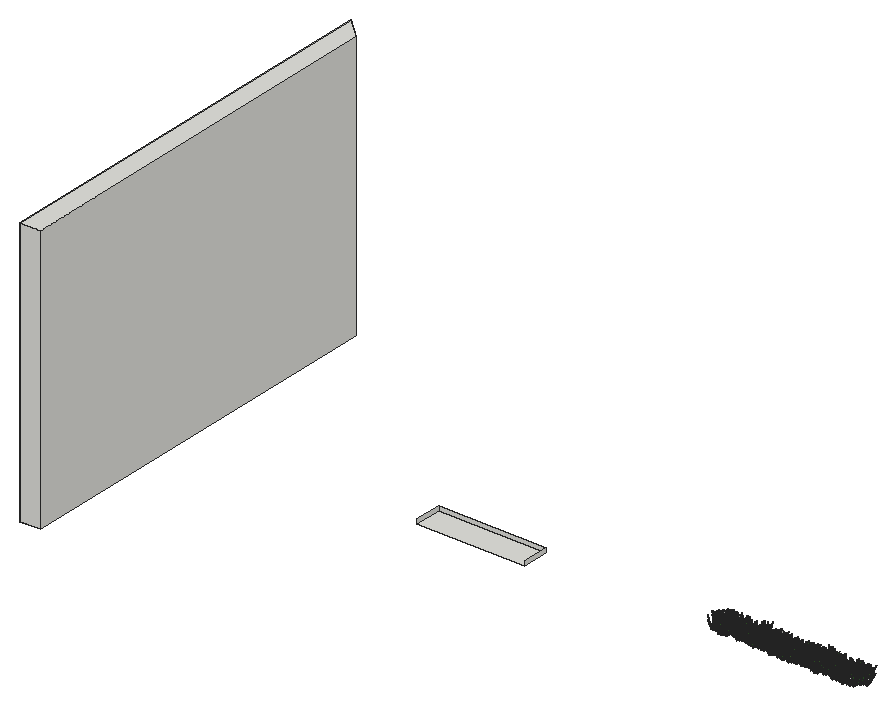
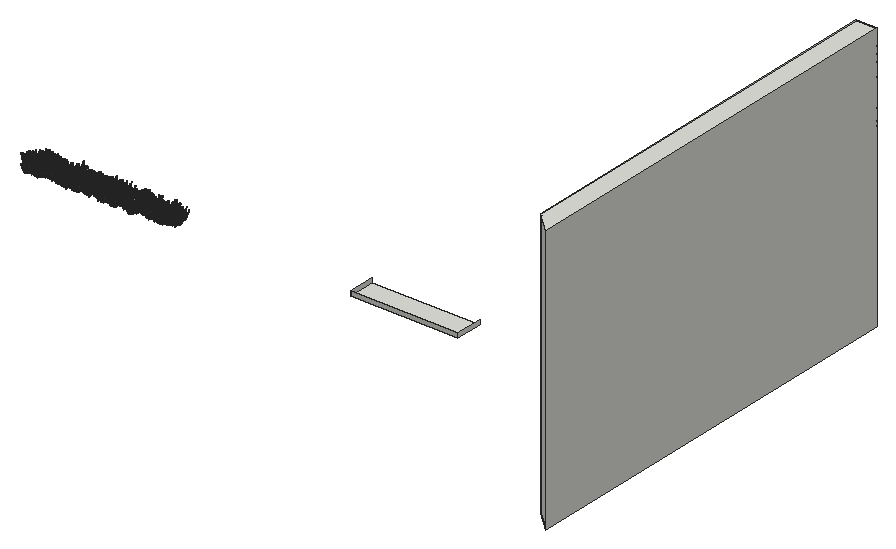
# SketchUp Ruby script. Lengths in inches.
U = 1.inch
M = Sketchup.active_model
def pt(a) = Geom::Point3d.new(a.map { |v| v * U })
def face(e, loops, mat)
  f = e.add_face(loops[0].map { |a| pt(a) })
  loops[1..].each { |l| e.add_face(l.map { |a| pt(a) }).erase! }
  f.material = f.back_material = mat if mat
  f
end
# faces: each face lists its corners as indices into pts; further lists are holes
def faces(e, pts, list, mat = nil) = list.each { |f| face(e, (f[0].is_a?(Array) ? f : [f]).map { |l| l.map { |i| pts[i] } }, mat) }
# xy, xz, yz: faces in a plane at the given z, y or x. An outline is a flat list of corners, or four numbers for a rectangle; further outlines are holes
def ring(l) = l.size == 4 ? [[l[0], l[1]], [l[2], l[1]], [l[2], l[3]], [l[0], l[3]]] : l.each_slice(2).to_a
def flat(e, list, mat, &to3) = list.each { |f| face(e, (f[0].is_a?(Array) ? f : [f]).map { |l| ring(l).map { |u, v| to3.(u, v) } }, mat) }
def xy(e, z, list, mat = nil) = flat(e, list, mat) { |x, y| [x, y, z] }
def xz(e, y, list, mat = nil) = flat(e, list, mat) { |x, z| [x, y, z] }
def yz(e, x, list, mat = nil) = flat(e, list, mat) { |y, z| [x, y, z] }
def lines(e, pts, list) = list.each { |a, b| e.add_line(pt(pts[a]), pt(pts[b])) }
# prism: a flat outline (further loops are holes) pulled along v
def prism(e, loops, v, mat = nil)
  f = face(e, loops, mat); d = Geom::Vector3d.new(v.map { |x| x * U })
  f.pushpull(f.normal.samedirection?(d) ? d.length : -d.length)
end
def box(e, o, s, mat = nil) = prism(e, [[o, [o[0] + s[0], o[1], o[2]], [o[0] + s[0], o[1] + s[1], o[2]], [o[0], o[1] + s[1], o[2]]]], [0, 0, s[2]], mat)
def at(x, y, z, deg = 0) = Geom::Transformation.translation(pt([x, y, z])) * Geom::Transformation.rotation(ORIGIN, Z_AXIS, deg.degrees)
def axes(o, x, y, z) = Geom::Transformation.new([*x, 0, *y, 0, *z, 0, *pt(o).to_a, 1])
def part(name) = M.definitions.add(name)
# library, detail: a bought-in or finely detailed component or shape, given as its bounding box
def library(name, o, s) = part(name).tap { |d| box(d.entities, o, s) }
def detail(e, o, s) = box(e.add_group.entities, o, s)
def put(e, d, t, mat = nil) = e.add_instance(d, t).tap { |i| i.material = mat if mat }
def group(e, t, mat = nil) = e.add_group.tap { |g| g.transformation = t; g.material = mat if mat }.entities
root = M.entities
M.materials.add("Material1").color = [58, 110, 58]
M.materials.add("Material10").color = [48, 100, 38]
M.materials.add("Material3").color = [68, 110, 58]
M.materials.add("Material4").color = [48, 90, 38]
M.materials.add("Material5").color = [68, 110, 48]
M.materials.add("Material6").color = [48, 90, 48]
M.materials.add("Material8").color = [58, 90, 38]
M.materials.add("Material9").color = [68, 100, 58]
c1 = part("grass00")
p = [[-0.6875,0.15,0],[-0.56,0.08,5.52],[-0.04,0.03,2.76],[0.48,-0.02,0],[0.35,-0.02,5.52],[-0.1,-0.14,5.52],
  [-0.12,0.65,8.37],[-0.42,0.65,8.37]]
faces(c1.entities,p,[[0,1,2,3],[3,2,4],[1,5,2],[5,4,2],[1,6,5],[4,5,6],[7,6,1]])
c2 = part("Group16\#1")
put(c2.entities,c1,axes([1.44,-0.61,-0.01],[0.05352,0.12609,0],[-0.10704,0.04543,0.07239],[0.06664,-0.02828,0.11628]),"Material6")
put(c2.entities,c1,axes([0.76,-0.15,-0.01],[0.04676,0.24062,0],[-0.23162,0.04501,0.06642],[0.0652,-0.01267,0.23595]),"Material3")
put(c2.entities,c1,axes([0.79,0.01,-0.01],[-0.00606,0.34651,0],[-0.34381,-0.00602,0.0432],[0.04319,0.00076,0.34386]))
put(c2.entities,c1,axes([1,0.23,-0.01],[-0.07192,0.31144,0],[-0.28722,-0.06632,0.1236],[0.12043,0.02781,0.29478]),"Material5")
put(c2.entities,c1,axes([1.66,0.77,-0.01],[-0.13828,0.29651,0],[-0.21551,-0.1005,0.22471],[0.20365,0.09498,0.23779]),"Material10")
put(c2.entities,c1,axes([0.6875,0.52,-0.01],[-0.18126,0.24051,0],[-0.22746,-0.17142,0.09788],[0.07817,0.05891,0.28481]),"Material5")
put(c2.entities,c1,axes([0.68,0.78,-0.01],[-0.215,0.18688,0],[-0.12385,-0.14248,0.21334],[0.13995,0.16101,0.18878]),"Material3")
put(c2.entities,c1,axes([0.56,1,-0.01],[-0.13756,0.07624,0],[-0.06159,-0.11112,0.0927],[0.04494,0.08108,0.12705]),"Material5")
put(c2.entities,c1,axes([0.2,0.64,-0.01],[-0.23729,0.07254,0],[-0.05711,-0.18681,0.153],[0.04473,0.14632,0.19535]),"Material10")
put(c2.entities,c1,axes([0.0625,0.72,-0.01],[-0.28874,0.02525,0],[-0.02179,-0.24916,0.14647],[0.01276,0.14591,0.25012]),"Material3")
put(c2.entities,c1,axes([-0.08,0.62,-0.01],[-0.34089,-0.04187,0],[0.03255,-0.26504,0.216],[-0.02633,0.21439,0.26703]),"Material10")
put(c2.entities,c1,axes([-0.34,0.98,-0.01],[-0.14314,-0.0493,0],[0.04397,-0.12769,0.06843],[-0.02228,0.0647,0.13505]),"Material10")
put(c2.entities,c1,axes([-0.87,1.45,-0.01],[-0.23488,-0.14114,0],[0.13761,-0.22901,0.06087],[-0.03135,0.05217,0.26717]))
put(c2.entities,c1,axes([-0.72,0.77,-0.01],[-0.14208,-0.13251,0],[0.07209,-0.0773,0.16301],[-0.11118,0.11922,0.1057]),"Material10")
put(c2.entities,c1,axes([-0.62,0.43,-0.01],[-0.14845,-0.21203,0],[0.18654,-0.13061,0.12304],[-0.10079,0.07057,0.22772]),"Material3")
put(c2.entities,c1,axes([-0.68,0.29,-0.01],[-0.13639,-0.32136,0],[0.31723,-0.13464,0.05579],[-0.05136,0.0218,0.34462]),"Material4")
put(c2.entities,c1,axes([-0.64,0.125,-0.01],[-0.0458,-0.23569,0],[0.22124,-0.043,0.08276],[-0.08124,0.01579,0.22538]),"Material1")
put(c2.entities,c1,axes([-1.6,-0.03,-0.01],[0.00576,-0.32897,0],[0.27526,0.00482,0.18018],[-0.18015,-0.00315,0.2753]),"Material5")
put(c2.entities,c1,axes([-1.36,-0.31,-0.01],[0.05718,-0.24765,0],[0.18172,0.04196,0.17267],[-0.16825,-0.03885,0.1865]),"Material10")
put(c2.entities,c1,axes([-1.54,-0.72,-0.01],[0.06537,-0.14017,0],[0.13555,0.06321,0.03939],[-0.0357,-0.01665,0.14956]))
put(c2.entities,c1,axes([-1.19,-0.9,-0.01],[0.09597,-0.12735,0],[0.11214,0.08451,0.07557],[-0.06035,-0.04548,0.14042]),"Material9")
put(c2.entities,c1,axes([-0.47,-0.54,-0.01],[0.11588,-0.10072,0],[0.0618,0.0711,0.12124],[-0.07953,-0.0915,0.0942]))
put(c2.entities,c1,axes([-0.47,-0.84,-0.01],[0.11927,-0.0661,0],[0.06603,0.11913,0.00646],[-0.00313,-0.00565,0.13621]),"Material5")
put(c2.entities,c1,axes([-0.38,-1.24,-0.01],[0.28037,-0.08571,0],[0.0618,0.20215,0.20315],[-0.05939,-0.19428,0.21139]),"Material9")
put(c2.entities,c1,axes([-0.06,-0.66,-0.01],[0.22719,-0.01987,0],[0.01247,0.14255,0.17758],[-0.01547,-0.17691,0.1431]),"Material8")
put(c2.entities,c1,axes([0.11,-0.89,-0.01],[0.14882,0.01828,0],[-0.01058,0.08611,0.12229],[0.01491,-0.12138,0.08676]),"Material6")
put(c2.entities,c1,axes([0.25,-0.72,-0.01],[0.20481,0.07053,0],[-0.06206,0.18022,0.10291],[0.03351,-0.0973,0.1906]),"Material6")
put(c2.entities,c1,axes([0.85,-1.42,-0.01],[0.16481,0.09904,0],[-0.09472,0.15762,0.05616],[0.02893,-0.04814,0.18389]),"Material5")
put(c2.entities,c1,axes([1.01,-1.09,-0.01],[0.21858,0.20385,0],[-0.17495,0.1876,0.15339],[0.10462,-0.11218,0.25652]),"Material10")
put(c2.entities,c1,axes([1.01,-0.71,-0.01],[0.08733,0.12473,0],[-0.06445,0.04512,0.13037],[0.1068,-0.07477,0.07867]),"Material6")
c3 = part("Group15\#1")
put(c3.entities,c2,at(0,0,0))
c4 = part("3darcstudiotree_grass00\#1")
put(c4.entities,c3,at(0,0,0))
xy(root,0,[[138.47,142.5,186.47,154.5]])
xz(root,154.5,[[138.47,0,186.47,2]])
yz(root,138.47,[[142.5,0,154.5,2]])
yz(root,186.47,[[142.5,0,154.5,2]])
put(root,c4,axes([328.01,147.54,0.25],[-0.99812,-0.23597,0],[0.29966,-0.87317,-0.03955],[0.01934,-0.05634,1.95202]))
put(root,c4,axes([303.16,147.6,0.25],[-0.99427,-0.5448,0],[0.56102,-0.70534,-0.0411],[0.03193,-0.04014,1.43569]))
put(root,c4,axes([325.42,147.52,0.25],[-1.23292,0.07319,0],[-0.09013,-1.04602,-0.06114],[-0.006,-0.06962,1.73764]))
put(root,c4,axes([329.43,147.77,0.25],[1.07781,0.18938,0],[-0.2093,0.82062,-0.03259],[-0.01079,0.04231,1.61556]))
put(root,c4,axes([293.99,147.58,0.25],[0.51316,0.9034,0],[-0.96575,0.37791,-0.03917],[-0.05959,0.02332,1.79585]))
put(root,c4,axes([321.9,147.76,0.25],[-0.54141,-0.69646,0],[0.787,-0.42147,-0.04434],[0.0525,-0.02812,1.31982]))
put(root,c4,axes([313.53,147.49,0.25],[-0.21956,0.99901,0],[-1.27509,-0.19305,-0.02378],[-0.03535,-0.00535,1.95907]))
put(root,c4,axes([298.41,147.61,0.25],[-0.29595,0.95829,0],[-1.17706,-0.25043,-0.05431],[-0.07294,-0.01552,1.6847]))
put(root,c4,axes([270.6875,147.76,0.25],[-0.64666,0.77516,0],[-0.79891,-0.45913,-0.03104],[-0.04689,-0.02695,1.78553]))
put(root,c4,axes([313.62,148.16,0.25],[1.22362,0.01748,0],[-0.01942,0.93658,-0.04862],[-0.00103,0.04974,1.39123]))
put(root,c4,axes([285.41,148.17,0.25],[-0.14791,-0.94502,0],[0.91047,-0.09817,-0.04034],[0.06426,-0.00693,1.47504]))
put(root,c4,axes([278.49,148.28,0.25],[-0.53102,-0.66775,0],[0.76975,-0.4217,-0.03406],[0.05336,-0.02923,1.73123]))
put(root,c4,axes([289.31,148.46,0.25],[0.95354,-0.47305,0],[0.61642,0.85599,-0.05659],[0.03982,0.0553,1.64805]))
put(root,c4,axes([317.27,148.26,0.25],[0.69662,0.57833,0],[-0.72973,0.60553,-0.04694],[-0.05459,0.0453,1.69685]))
put(root,c4,axes([283.84,148.47,0.25],[-0.01645,-0.79546,0],[1.12073,-0.01596,-0.0405],[0.06828,-0.00097,1.89003]))
put(root,c4,axes([307.7,148.16,0.25],[-0.67385,0.62223,0],[-0.80238,-0.59862,-0.05045],[-0.05166,-0.03854,1.48531]))
put(root,c4,axes([296.36,148.12,0.25],[-1.1835,0.3706,0],[-0.45111,-0.99242,-0.03096],[-0.01538,-0.03383,1.79846]))
put(root,c4,axes([283.37,148.31,0.25],[-0.12789,0.83027,0],[-1.23138,-0.13067,-0.0277],[-0.0416,-0.00441,1.87956]))
put(root,c4,axes([295.22,148.47,0.25],[0.68284,0.56041,0],[-0.63274,0.53112,-0.02576],[-0.03793,0.03184,1.88472]))
put(root,c4,axes([310.07,148.73,0.25],[0.39676,-0.79081,0],[0.95001,0.32835,-0.04485],[0.06401,0.02212,1.59096]))
put(root,c4,axes([322.74,148.87,0.25],[0.81664,-0.78547,0],[0.80725,0.57818,-0.04774],[0.06475,0.04638,1.91023]))
put(root,c4,axes([298.375,148.73,0.25],[0.72037,0.53225,0],[-0.78121,0.72839,-0.03405],[-0.03196,0.0298,1.65877]))
put(root,c4,axes([267.24,148.87,0.25],[1.1348,0.18325,0],[-0.22931,0.97826,-0.03864],[-0.01139,0.04857,1.85268]))
put(root,c4,axes([323.75,148.72,0.25],[0.82375,0.73045,0],[-0.83513,0.6488,-0.05678],[-0.04846,0.03764,1.337]))
put(root,c4,axes([287.74,148.83,0.25],[-0.54485,-0.78399,0],[0.98958,-0.47378,-0.05686],[0.05654,-0.02707,1.31145]))
put(root,c4,axes([327.1,148.96,0.25],[0.55568,-0.81643,0],[0.99319,0.46568,-0.05349],[0.08034,0.03767,1.96798]))
put(root,c4,axes([272.17,148.61,0.25],[-0.33702,0.82532,0],[-1.09541,-0.30816,-0.05878],[-0.06687,-0.01881,1.38915]))
put(root,c4,axes([312.09,149,0.25],[0.98512,-0.69325,0],[0.69961,0.68488,-0.04452],[0.05205,0.05095,1.95574]))
put(root,c4,axes([308.19,148.69,0.25],[0.10661,0.83198,0],[-1.11243,0.0982,-0.05804],[-0.07208,0.00636,1.39706]))
put(root,c4,axes([304.56,148.93,0.25],[-0.23365,-0.75886,0],[0.96416,-0.20451,-0.03508],[0.06527,-0.01385,1.91126]))
put(root,c4,axes([328.56,148.91,0.25],[-0.34662,-0.71179,0],[1.07984,-0.36226,-0.05241],[0.06977,-0.02341,1.67241]))
put(root,c4,axes([291.52,148.86,0.25],[-0.96963,-0.34021,0],[0.44355,-0.87089,-0.0473],[0.02319,-0.04554,1.43445]))
put(root,c4,axes([299.84,148.98,0.25],[0.68299,0.59104,0],[-0.74364,0.59199,-0.02632],[-0.036,0.02866,1.95302]))
put(root,c4,axes([325.33,148.93,0.25],[-0.68826,0.85119,0],[-0.91752,-0.51109,-0.03945],[-0.04757,-0.0265,1.6047]))
g1 = group(root,at(28.97,57,0))
prism(g1,[[[0,184.95,0],[9,176.76,0],[9,0,0],[0,0,0]]],[0,0,120])
put(root,c4,axes([294.65,149.54,0.25],[-0.53689,-0.61201,0],[0.94056,-0.56841,-0.06067],[0.0763,-0.04611,1.80988]))
put(root,c4,axes([309.77,149.41,0.25],[-1.07879,-0.10115,0],[0.14303,-1.0509,-0.03054],[0.00494,-0.03632,1.83699]))
put(root,c4,axes([299.68,149.43,0.25],[-1.04284,0.49546,0],[-0.47914,-0.69475,-0.03218],[-0.02748,-0.03984,1.65786]))
put(root,c4,axes([330.25,149.6,0.25],[1.09397,0.55734,0],[-0.51476,0.69606,-0.0354],[-0.03655,0.04943,1.94218]))
put(root,c4,axes([307.6,149.45,0.25],[-0.41932,0.80562,0],[-1.07652,-0.38601,-0.05011],[-0.06628,-0.02377,1.6899]))
put(root,c4,axes([297.53,149.85,0.25],[0.12612,-1.06653,0],[1.18822,0.09679,-0.05803],[0.06333,0.00516,1.30918]))
put(root,c4,axes([280.05,149.79,0.25],[-0.22458,-0.91209,0],[1.19453,-0.20262,-0.03636],[0.04783,-0.00811,1.63697]))
put(root,c4,axes([302.12,149.49,0.25],[-0.75397,0.48628,0],[-0.78378,-0.83717,-0.03993],[-0.03716,-0.03969,1.9372]))
put(root,c4,axes([328.16,149.59,0.25],[0.04239,0.95828,0],[-1.1135,0.03393,-0.05084],[-0.07764,0.00237,1.70302]))
put(root,c4,axes([272.34,150.02,0.25],[0.10246,-1.02082,0],[1.01002,0.06984,-0.04948],[0.08579,0.00593,1.76318]))
put(root,c4,axes([324.16,149.82,0.25],[0.47136,0.68129,0],[-1.02177,0.48701,-0.0451],[-0.06422,0.03061,1.93445]))
put(root,c4,axes([278.51,149.88,0.25],[1.07292,0.6068,0],[-0.64763,0.78887,-0.06012],[-0.03975,0.04841,1.3502]))
put(root,c4,axes([276.41,150.08,0.25],[0.9139,-0.00536,0],[0.00825,0.96856,-0.0442],[0.00036,0.04202,1.33678]))
put(root,c4,axes([327.1,150.19,0.25],[0.05371,-0.98895,0],[0.90708,0.03394,-0.03915],[0.08404,0.00314,1.95085]))
put(root,c4,axes([293.46,149.9,0.25],[-0.98303,0.21061,0],[-0.25379,-0.81607,-0.03018],[-0.01473,-0.04737,1.98332]))
put(root,c4,axes([275.85,150.19,0.25],[-0.66708,-0.80453,0],[0.96955,-0.55381,-0.05298],[0.05473,-0.03126,1.4759]))
put(root,c4,axes([301.52,149.99,0.25],[-0.18994,0.90501,0],[-0.90116,-0.13029,-0.03897],[-0.07458,-0.01078,1.77692]))
put(root,c4,axes([320.96,150.07,0.25],[-0.1834,0.89621,0],[-1.14917,-0.162,-0.06003],[-0.09372,-0.01321,1.84592]))
put(root,c4,axes([304.5,150.12,0.25],[-0.5195,0.6578,0],[-0.76531,-0.41638,-0.04],[-0.05333,-0.02902,1.45882]))
put(root,c4,axes([273.39,150.26,0.25],[0.61609,0.66998,0],[-0.73554,0.46596,-0.04536],[-0.075,0.04751,1.92466]))
put(root,c4,axes([296.93,150.66,0.25],[0.83761,-0.62775,0],[0.72957,0.67062,-0.04418],[0.04566,0.04197,1.67893]))
put(root,c4,axes([287,150.72,0.25],[0.25933,-0.91645,0],[1.15367,0.2249,-0.04288],[0.06004,0.0117,1.70449]))
put(root,c4,axes([269.16,150.95,0.25],[0.27626,-0.85424,0],[1.12911,0.25155,-0.05256],[0.06907,0.01539,1.59089]))
put(root,c4,axes([327.875,151.01,0.25],[0.88851,-0.34477,0],[0.5209,0.92478,-0.04906],[0.03091,0.05488,1.82977]))
put(root,c4,axes([275.09,150.62,0.25],[-0.8401,0.75363,0],[-0.79268,-0.60873,-0.0352],[-0.03888,-0.02986,1.62511]))
put(root,c4,axes([278.49,151.03,0.25],[0.16464,-0.97874,0],[0.9194,0.10654,-0.0384],[0.06278,0.00728,1.53253]))
put(root,c4,axes([308.42,150.87,0.25],[-0.99278,-0.20343,0],[0.28077,-0.94395,-0.03453],[0.01024,-0.03443,1.44935]))
put(root,c4,axes([305.66,151.04,0.25],[1.12356,0.40901,0],[-0.43138,0.81634,-0.04488],[-0.03317,0.06278,1.97665]))
put(root,c4,axes([322.75,151.18,0.25],[0.92045,-0.04045,0],[0.04941,0.77465,-0.02933],[0.00328,0.05139,1.97542]))
put(root,c4,axes([332.51,151.09,0.25],[-0.88862,-0.44543,0],[0.46637,-0.64095,-0.04514],[0.04258,-0.05852,1.64638]))
put(root,c4,axes([313.22,151.33,0.25],[0.78359,-0.40268,0],[0.59064,0.79179,-0.03178],[0.02468,0.03309,1.65559]))
put(root,c4,axes([306.62,151.4,0.25],[0.8358,-0.48818,0],[0.70624,0.83298,-0.04926],[0.04459,0.0526,1.93034]))
put(root,c4,axes([273.78,151.4,0.25],[-0.03414,-1.03795,0],[1.29278,-0.0293,-0.06757],[0.09119,-0.00207,1.74608]))
put(root,c4,axes([299.12,151.54,0.25],[0.34855,-0.69685,0],[0.94344,0.32508,-0.03248],[0.04735,0.01631,1.61223]))
put(root,c4,axes([297.52,151.3,0.25],[0.31087,0.78907,0],[-1.06486,0.28901,-0.05705],[-0.07395,0.02007,1.52794]))
put(root,c4,axes([310.57,151.23,0.25],[-0.6188,0.78676,0],[-1.0343,-0.56042,-0.02867],[-0.03468,-0.01879,1.78429]))
put(root,c4,axes([291.51,151.39,0.25],[0.33625,0.70775,0],[-0.90299,0.29554,-0.04901],[-0.07739,0.02533,1.64754]))
put(root,c4,axes([280.81,151.34,0.25],[-0.26408,0.8051,0],[-1.23394,-0.27883,-0.06593],[-0.07968,-0.018,1.60187]))
put(root,c4,axes([329.89,151.37,0.25],[-0.30442,0.74755,0],[-0.92944,-0.26074,-0.04196],[-0.06575,-0.01845,1.62262]))
put(root,c4,axes([271.84,151.5,0.25],[-1.09069,-0.34377,0],[0.40445,-0.88401,-0.04397],[0.02642,-0.05775,1.92843]))
put(root,c4,axes([321,151.49,0.25],[-0.85998,-0.29123,0],[0.416,-0.84626,-0.03312],[0.02206,-0.04487,1.94116]))
put(root,c4,axes([316.6,151.45,0.25],[-1.1185,0.45043,0],[-0.55571,-0.95063,-0.06144],[-0.02869,-0.04908,1.3618]))
put(root,c4,axes([271.78,151.97,0.25],[1.06027,-0.42495,0],[0.42484,0.73023,-0.04306],[0.03738,0.06425,1.95064]))
put(root,c4,axes([304.42,152.15,0.25],[1.00798,-0.05122,0],[0.0779,1.05614,-0.0507],[0.00404,0.05482,1.66388]))
put(root,c4,axes([331.03,152.22,0.25],[1.23576,-0.22266,0],[0.25493,0.97468,-0.03342],[0.01129,0.04317,1.91382]))
put(root,c4,axes([267.57,152.28,0.25],[-0.57718,-0.85275,0],[0.96086,-0.44803,-0.0488],[0.05124,-0.02389,1.32723]))
put(root,c4,axes([291.87,152.28,0.25],[1.16828,0.38492,0],[-0.38794,0.81115,-0.04113],[-0.01985,0.0415,1.37498]))
put(root,c4,axes([301.21,152.04,0.25],[-0.23065,0.90019,0],[-1.12909,-0.1993,-0.02719],[-0.04135,-0.0073,1.79436]))
put(root,c4,axes([287.04,152.43,0.25],[1.13745,-0.3405,0],[0.42127,0.96946,-0.06016],[0.02508,0.05772,1.52593]))
put(root,c4,axes([285.9375,152.08,0.25],[0.17726,0.99007,0],[-0.98286,0.12123,-0.03328],[-0.05081,0.00627,1.53387]))
put(root,c4,axes([312.69,152.18,0.25],[0.39858,0.80872,0],[-1.17659,0.39948,-0.06498],[-0.0914,0.03103,1.93183]))
put(root,c4,axes([322.22,152.51,0.25],[0.80451,-0.53933,0],[0.65383,0.6719,-0.03491],[0.039,0.04008,1.84986]))
put(root,c4,axes([273.73,152.58,0.25],[0.91031,-0.47162,0],[0.58028,0.7716,-0.03499],[0.03194,0.04247,1.88939]))
put(root,c4,axes([266.5,152.17,0.25],[-0.91774,0.55562,0],[-0.69789,-0.79413,-0.03459],[-0.03172,-0.03609,1.84283]))
put(root,c4,axes([297.75,152.46,0.25],[-0.75496,-0.74499,0],[0.86531,-0.60409,-0.04595],[0.05448,-0.03803,1.75181]))
put(root,c4,axes([283.95,152.55,0.25],[-0.38021,-0.89194,0],[0.97708,-0.28693,-0.03351],[0.0515,-0.01512,1.68972]))
put(root,c4,axes([329.42,152.65,0.25],[0.32176,-0.95016,0],[1.10359,0.25745,-0.04021],[0.05861,0.01367,1.73573]))
put(root,c4,axes([296.18,152.56,0.25],[1.05579,0.41983,0],[-0.50742,0.87908,-0.04599],[-0.0231,0.04002,1.36526]))
put(root,c4,axes([310.61,152.73,0.25],[0.72155,-0.65742,0],[0.95802,0.72436,-0.04921],[0.04681,0.03539,1.66765]))
put(root,c4,axes([316.21,152.57,0.25],[-0.58412,-0.61774,0],[0.94474,-0.61542,-0.04646],[0.05533,-0.03604,1.81816]))
put(root,c4,axes([328.8,152.71,0.25],[0.91357,-0.05751,0],[0.08718,0.95406,-0.06006],[0.00603,0.066,1.53056]))
put(root,c4,axes([306.7,152.47,0.25],[-1.1695,-0.19764,0],[0.24295,-0.99036,-0.03896],[0.01129,-0.04601,1.76791]))
put(root,c4,axes([271.19,152.46,0.25],[-0.663,0.54245,0],[-0.85594,-0.7207,-0.05994],[-0.05232,-0.04405,1.51606]))
put(root,c4,axes([295.08,152.77,0.25],[-1.03221,-0.54752,0],[0.64555,-0.83839,-0.05584],[0.04863,-0.06316,1.93872]))
put(root,c4,axes([281.5,152.6,0.25],[-0.16604,1.03098,0],[-0.98673,-0.10948,-0.04319],[-0.0805,-0.00893,1.87209]))
put(root,c4,axes([298.99,152.65,0.25],[-0.18531,1.05276,0],[-0.99477,-0.12063,-0.03578],[-0.04722,-0.00573,1.34076]))
put(root,c4,axes([318.11,153.125,0.25],[1.07701,0.22261,0],[-0.2539,0.84626,-0.04825],[-0.0162,0.05398,1.45973]))
put(root,c4,axes([266.46,153.29,0.25],[0.84889,0.27567,0],[-0.45867,0.97301,-0.03882],[-0.01752,0.03717,1.55956]))
put(root,c4,axes([268,153.16,0.25],[0.76375,0.58285,0],[-0.72277,0.65246,-0.04265],[-0.05136,0.04637,1.90027]))
put(root,c4,axes([323.71,153.26,0.25],[-0.86123,-0.76787,0],[0.702,-0.54241,-0.04944],[0.06067,-0.04688,1.60821]))
put(root,c4,axes([299.93,153.375,0.25],[1.12005,-0.34432,0],[0.32915,0.73759,-0.03178],[0.02101,0.04709,1.80429]))
put(root,c4,axes([318.8,153.35,0.25],[0.77918,0.46115,0],[-0.63013,0.73346,-0.03635],[-0.02744,0.03194,1.41103]))
put(root,c4,axes([315.17,153.55,0.25],[0.12485,-1.01104,0],[1.23512,0.10507,-0.06373],[0.07671,0.00653,1.50237]))
put(root,c4,axes([325.78,153.39,0.25],[0.64935,0.62902,0],[-0.96898,0.68911,-0.05975],[-0.04946,0.03517,1.3909]))
put(root,c4,axes([283.12,153.46,0.25],[-0.61486,-0.67806,0],[0.75305,-0.47042,-0.02546],[0.04194,-0.0262,1.94365]))
put(root,c4,axes([306.99,153.57,0.25],[1.15462,-0.15811,0],[0.16177,0.81384,-0.03976],[0.01148,0.05773,1.7619]))
put(root,c4,axes([289.06,153.63,0.25],[-0.52106,-0.71154,0],[0.80489,-0.40605,-0.04312],[0.07514,-0.0379,1.92045]))
put(root,c4,axes([269.08,153.41,0.25],[-0.69174,0.87827,0],[-0.85626,-0.4646,-0.05029],[-0.08186,-0.04441,1.98932]))
put(root,c4,axes([326.82,153.82,0.25],[0.40583,-0.83092,0],[1.1915,0.4009,-0.03495],[0.04634,0.01559,1.83937]))
put(root,c4,axes([279.54,153.83,0.25],[0.03989,-0.78048,0],[1.24616,0.04388,-0.04061],[0.05562,0.00196,1.70991]))
put(root,c4,axes([291.88,153.76,0.25],[1.02267,0.32459,0],[-0.37336,0.81039,-0.02441],[-0.01644,0.03569,1.97124]))
put(root,c4,axes([272.06,153.56,0.25],[0.03285,0.80579,0],[-1.22967,0.03453,-0.06181],[-0.08889,0.0025,1.77032]))
put(root,c4,axes([331.1,153.91,0.25],[0.6129,-0.7876,0],[1.01266,0.54288,-0.0579],[0.07459,0.03998,1.84885]))
put(root,c4,axes([305.51,153.92,0.25],[1.12908,0.05835,0],[-0.06338,0.84486,-0.04181],[-0.00497,0.06627,1.95138]))
put(root,c4,axes([304.45,153.74,0.25],[-1.13599,0.20569,0],[-0.23567,-0.89663,-0.03649],[-0.01269,-0.04827,1.80375]))
put(root,c4,axes([300.97,153.84,0.25],[-0.87627,0.50999,0],[-0.57442,-0.67993,-0.04222],[-0.04259,-0.05042,1.75818]))
put(root,c4,axes([321.98,153.95,0.25],[-0.77794,0.56312,0],[-0.71742,-0.68277,-0.0546],[-0.06081,-0.05788,1.84968]))
put(root,c4,axes([308.12,154.04,0.25],[0.22597,0.91949,0],[-0.9349,0.15828,-0.03877],[-0.0772,0.01307,1.93915]))
put(root,c4,axes([277.16,153.98,0.25],[-0.68474,0.55059,0],[-0.81726,-0.70018,-0.02879],[-0.03,-0.0257,1.7592]))
put(root,c4,axes([291.53,154.4375,0.25],[0.5561,-0.60692,0],[1.02155,0.64481,-0.04371],[0.03815,0.02408,1.40723]))
put(root,c4,axes([269.4,154.42,0.25],[1.1087,0.48983,0],[-0.56089,0.87457,-0.02998],[-0.02338,0.03645,1.98098]))
put(root,c4,axes([286.17,154.62,0.25],[0.61935,-0.69322,0],[0.94107,0.57922,-0.03781],[0.03732,0.02297,1.4396]))
put(root,c4,axes([329.39,154.39,0.25],[0.29325,0.94894,0],[-1.11116,0.23656,-0.04684],[-0.05615,0.01195,1.41954]))
put(root,c4,axes([309.88,154.4,0.25],[0.12088,0.92692,0],[-1.25906,0.11311,-0.03135],[-0.03771,0.00339,1.53244]))
put(root,c4,axes([319.65,154.4375,0.25],[0.19911,0.81194,0],[-1.01825,0.17202,-0.02796],[-0.05135,0.00867,1.94708]))
put(root,c4,axes([313.14,154.53,0.25],[0.56819,0.58082,0],[-0.81333,0.54812,-0.04172],[-0.05517,0.03718,1.78477]))
put(root,c4,axes([315.07,154.68,0.25],[-0.61124,-0.75412,0],[0.98194,-0.54829,-0.0439],[0.04758,-0.02657,1.54604]))
put(root,c4,axes([324.13,154.75,0.25],[-0.551,-0.9345,0],[1.12732,-0.45791,-0.06506],[0.07959,-0.03233,1.70958]))
put(root,c4,axes([326.74,154.56,0.25],[-1.00692,-0.15209,0],[0.1808,-0.82461,-0.02729],[0.00905,-0.0413,1.8715]))
put(root,c4,axes([295.17,154.47,0.25],[-0.96869,0.62402,0],[-0.71,-0.75929,-0.03049],[-0.02804,-0.02998,1.73706]))
put(root,c4,axes([270.42,154.85,0.25],[1.06162,-0.22098,0],[0.21999,0.72808,-0.03452],[0.01731,0.05728,1.86367]))
put(root,c4,axes([283.1,154.96,0.25],[0.40604,-0.68535,0],[0.86838,0.35442,-0.04022],[0.07451,0.03041,1.99791]))
put(root,c4,axes([271.86,154.97,0.25],[0.87595,0.21429,0],[-0.34099,0.96021,-0.04213],[-0.01409,0.03968,1.42653]))
put(root,c4,axes([275.86,154.77,0.25],[0.32498,0.71712,0],[-0.97484,0.30434,-0.04913],[-0.0803,0.02507,1.81865]))
put(root,c4,axes([302.93,155.15,0.25],[1.12066,0.00691,0],[-0.00791,0.88387,-0.04293],[-0.00041,0.04534,1.35522]))
put(root,c4,axes([316.04,155.11,0.25],[-0.90107,-0.45582,0],[0.49292,-0.67128,-0.03312],[0.03112,-0.04237,1.70984]))
put(root,c4,axes([329.72,155.88,0.25],[-0.56595,-0.84976,0],[0.81458,-0.37374,-0.04183],[0.0585,-0.02684,1.48723]))
put(root,c4,axes([312.8,155.88,0.25],[0.94446,0.07549,0],[-0.09712,0.83701,-0.03978],[-0.00743,0.06406,1.9745]))
put(root,c4,axes([325.86,155.91,0.25],[0.97364,0.03456,0],[-0.04879,0.94689,-0.05798],[-0.00348,0.06756,1.60438]))
put(root,c4,axes([283.35,155.95,0.25],[-0.48002,-0.88518,0],[1.0357,-0.38692,-0.04331],[0.06566,-0.02453,1.88835]))
put(root,c4,axes([308.33,155.74,0.25],[-1.12816,-0.15626,0],[0.1793,-0.89178,-0.03361],[0.00782,-0.03892,1.54092]))
put(root,c4,axes([296.74,155.84,0.25],[-0.87392,-0.34377,0],[0.46155,-0.80831,-0.03887],[0.02264,-0.03965,1.46596]))
put(root,c4,axes([291.4375,155.77,0.25],[-1.07655,-0.01518,0],[0.02054,-1.00347,-0.03595],[0.00084,-0.04106,1.66434]))
